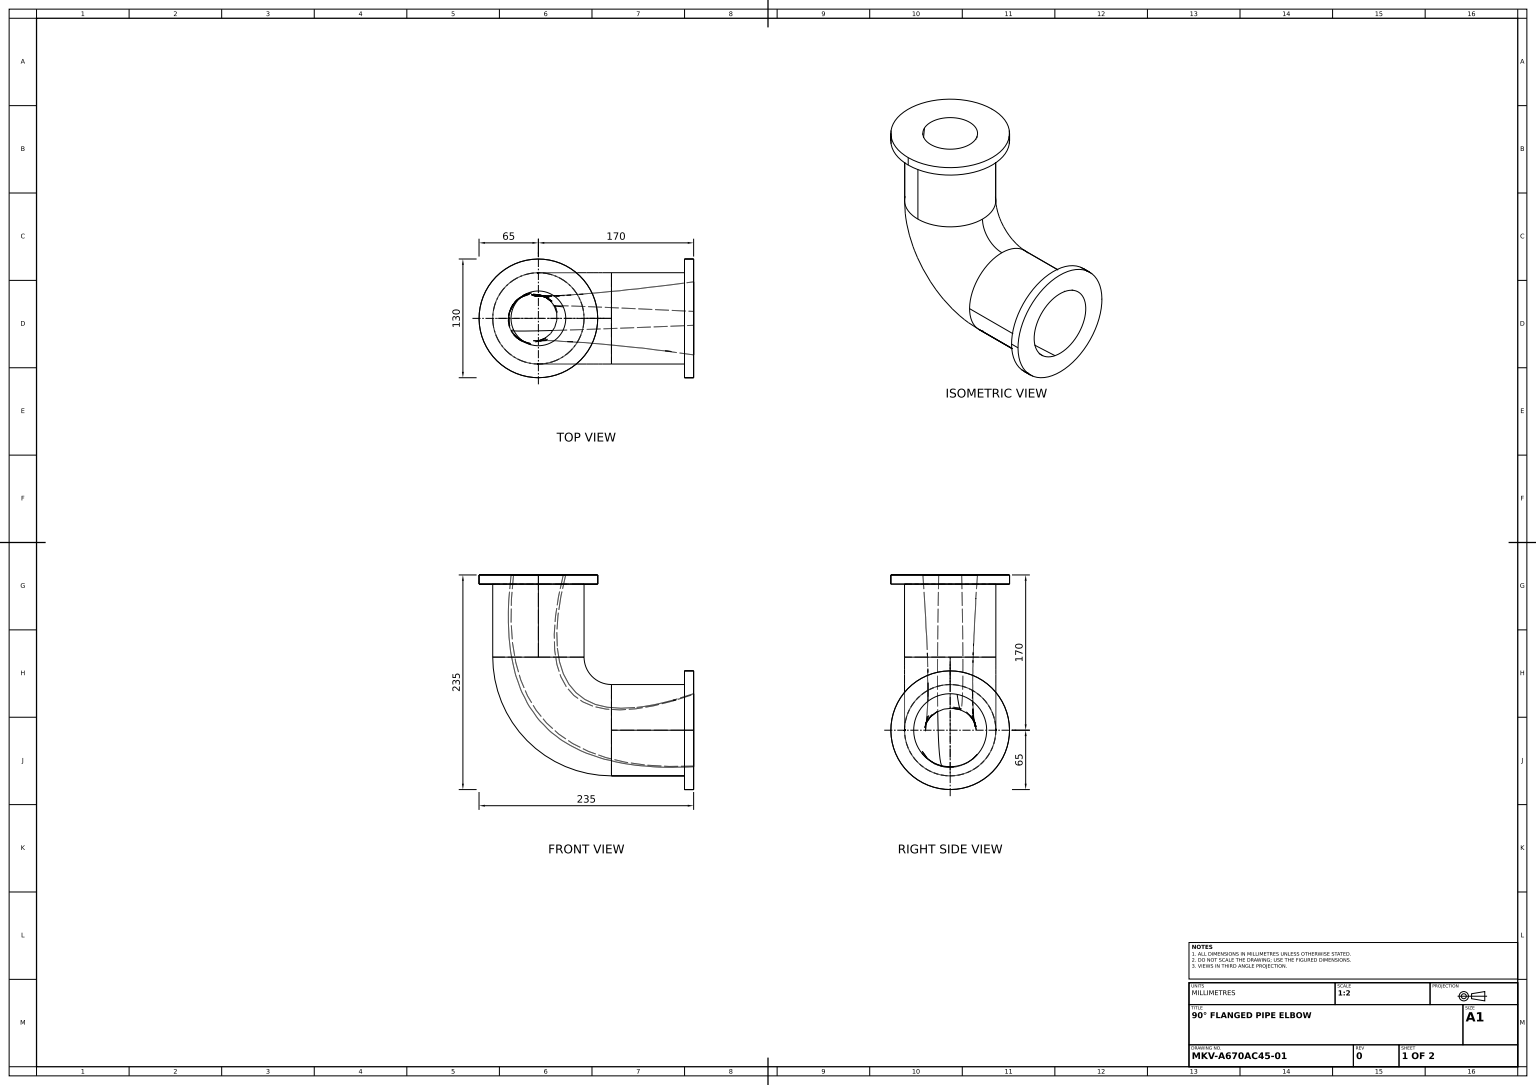
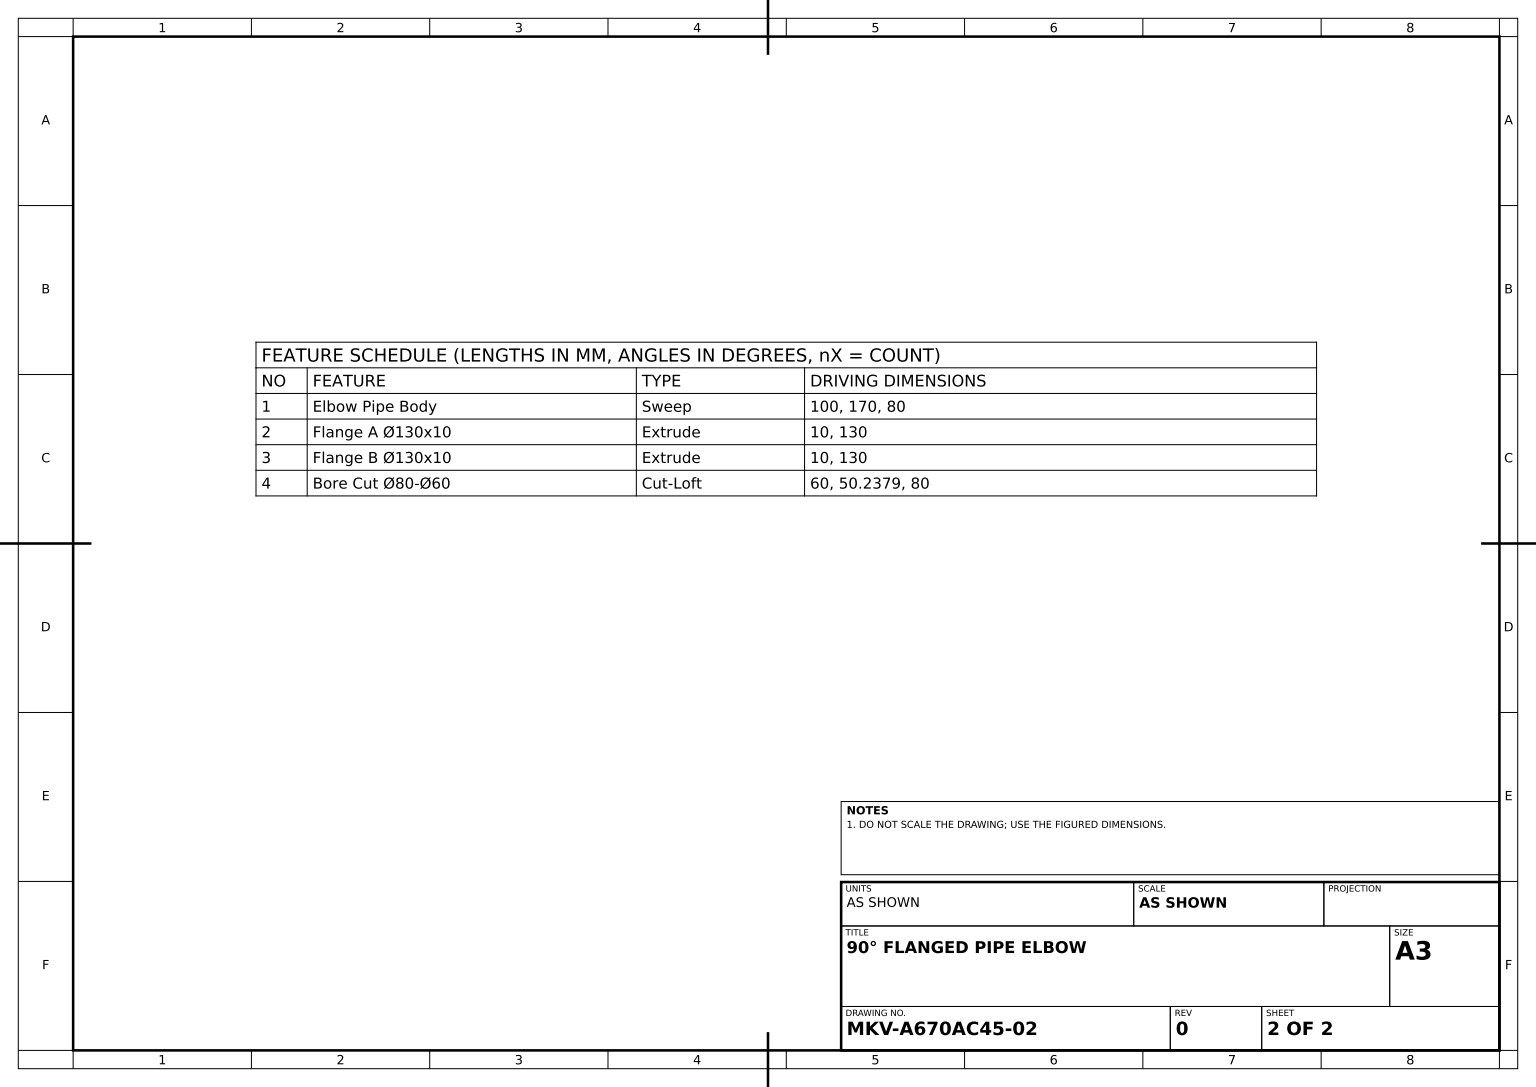
ISO-10303-21;
HEADER;
FILE_DESCRIPTION((''),'2;1');
FILE_NAME('','',(''),(''),'','','');
FILE_SCHEMA(('AUTOMOTIVE_DESIGN'));
ENDSEC;
DATA;
#1=APPLICATION_CONTEXT('');
#2=PRODUCT_CONTEXT('',#1,'mechanical');
#3=PRODUCT('','','',(#2));
#4=PRODUCT_DEFINITION_FORMATION('','',#3);
#5=PRODUCT_DEFINITION_CONTEXT('',#1,'design');
#6=PRODUCT_DEFINITION('','',#4,#5);
#7=PRODUCT_DEFINITION_SHAPE('','',#6);
#8=(LENGTH_UNIT()NAMED_UNIT(*)SI_UNIT(.MILLI.,.METRE.));
#9=(NAMED_UNIT(*)PLANE_ANGLE_UNIT()SI_UNIT($,.RADIAN.));
#10=(NAMED_UNIT(*)SI_UNIT($,.STERADIAN.)SOLID_ANGLE_UNIT());
#11=UNCERTAINTY_MEASURE_WITH_UNIT(LENGTH_MEASURE(1.E-05),#8,'distance_accuracy_value','');
#12=(GEOMETRIC_REPRESENTATION_CONTEXT(3)GLOBAL_UNCERTAINTY_ASSIGNED_CONTEXT((#11))GLOBAL_UNIT_ASSIGNED_CONTEXT((#8,#9,#10))REPRESENTATION_CONTEXT('',''));
#13=CARTESIAN_POINT('',(-170.,170.,65.));
#14=VERTEX_POINT('',#13);
#15=CARTESIAN_POINT('',(-170.,170.,-65.));
#16=VERTEX_POINT('',#15);
#17=CARTESIAN_POINT('',(-170.,170.,0.));
#18=DIRECTION('',(0.,1.,0.));
#19=DIRECTION('',(0.,0.,1.));
#20=AXIS2_PLACEMENT_3D('',#17,#18,#19);
#21=CIRCLE('',#20,65.);
#22=EDGE_CURVE('',#14,#16,#21,.T.);
#23=ORIENTED_EDGE('',*,*,#22,.T.);
#24=EDGE_CURVE('',#16,#14,#21,.T.);
#25=ORIENTED_EDGE('',*,*,#24,.T.);
#26=EDGE_LOOP('',(#23,#25));
#27=FACE_OUTER_BOUND('',#26,.T.);
#28=CARTESIAN_POINT('',(-197.232446,170.,12.585464));
#29=VERTEX_POINT('',#28);
#30=CARTESIAN_POINT('',(-142.767554,170.,-12.585464));
#31=VERTEX_POINT('',#30);
#32=CIRCLE('',#20,30.);
#33=EDGE_CURVE('',#29,#31,#32,.T.);
#34=ORIENTED_EDGE('',*,*,#33,.F.);
#35=EDGE_CURVE('',#31,#29,#32,.T.);
#36=ORIENTED_EDGE('',*,*,#35,.F.);
#37=EDGE_LOOP('',(#34,#36));
#38=FACE_BOUND('',#37,.T.);
#39=PLANE('',#20);
#40=ADVANCED_FACE('',(#27,#38),#39,.T.);
#41=CARTESIAN_POINT('',(-170.,160.,-65.));
#42=VERTEX_POINT('',#41);
#43=CARTESIAN_POINT('',(-170.,160.,65.));
#44=VERTEX_POINT('',#43);
#45=CARTESIAN_POINT('',(-170.,160.,0.));
#46=AXIS2_PLACEMENT_3D('',#45,#18,#19);
#47=CIRCLE('',#46,65.);
#48=EDGE_CURVE('',#42,#44,#47,.T.);
#49=ORIENTED_EDGE('',*,*,#48,.T.);
#50=VECTOR('',#18,1000.);
#51=LINE('',#43,#50);
#52=EDGE_CURVE('',#44,#14,#51,.T.);
#53=ORIENTED_EDGE('',*,*,#52,.T.);
#54=ORIENTED_EDGE('',*,*,#24,.F.);
#55=LINE('',#41,#50);
#56=EDGE_CURVE('',#42,#16,#55,.T.);
#57=ORIENTED_EDGE('',*,*,#56,.F.);
#58=EDGE_LOOP('',(#49,#53,#54,#57));
#59=FACE_OUTER_BOUND('',#58,.T.);
#60=CYLINDRICAL_SURFACE('',#46,65.);
#61=ADVANCED_FACE('',(#59),#60,.T.);
#62=ORIENTED_EDGE('',*,*,#22,.F.);
#63=ORIENTED_EDGE('',*,*,#52,.F.);
#64=EDGE_CURVE('',#44,#42,#47,.T.);
#65=ORIENTED_EDGE('',*,*,#64,.T.);
#66=ORIENTED_EDGE('',*,*,#56,.T.);
#67=EDGE_LOOP('',(#62,#63,#65,#66));
#68=FACE_OUTER_BOUND('',#67,.T.);
#69=ADVANCED_FACE('',(#68),#60,.T.);
#70=CARTESIAN_POINT('',(0.,39.272528,-7.593979));
#71=VERTEX_POINT('',#70);
#72=CARTESIAN_POINT('',(-159.156042,104.12626,-14.002019));
#73=CARTESIAN_POINT('',(-151.137946,15.902503,-14.565282));
#74=CARTESIAN_POINT('',(-63.977673,16.974613,-10.674363));
#75=B_SPLINE_CURVE_WITH_KNOTS('',3,(#30,#72,#73,#74,#70),.UNSPECIFIED.,.F.,.F.,(4,1,4),(0.,0.497690593,1.),.UNSPECIFIED.);
#76=EDGE_CURVE('',#31,#71,#75,.T.);
#77=ORIENTED_EDGE('',*,*,#76,.F.);
#78=ORIENTED_EDGE('',*,*,#35,.T.);
#79=CARTESIAN_POINT('',(0.,-39.272528,7.593979));
#80=VERTEX_POINT('',#79);
#81=CARTESIAN_POINT('',(-205.914144,96.731109,13.989567));
#82=CARTESIAN_POINT('',(-182.354184,-10.749397,14.577735));
#83=CARTESIAN_POINT('',(-74.425847,-42.78391,10.66191));
#84=B_SPLINE_CURVE_WITH_KNOTS('',3,(#28,#81,#82,#83,#79),.UNSPECIFIED.,.F.,.F.,(4,1,4),(0.,0.497690593,1.),.UNSPECIFIED.);
#85=EDGE_CURVE('',#29,#80,#84,.T.);
#86=ORIENTED_EDGE('',*,*,#85,.T.);
#87=CARTESIAN_POINT('',(0.,0.,0.));
#88=DIRECTION('',(1.,0.,0.));
#89=DIRECTION('',(0.,0.,-1.));
#90=AXIS2_PLACEMENT_3D('',#87,#88,#89);
#91=CIRCLE('',#90,40.);
#92=EDGE_CURVE('',#80,#71,#91,.T.);
#93=ORIENTED_EDGE('',*,*,#92,.T.);
#94=EDGE_LOOP('',(#77,#78,#86,#93));
#95=FACE_OUTER_BOUND('',#94,.T.);
#96=CARTESIAN_POINT('',(-142.420249,170.,-11.833964));
#97=CARTESIAN_POINT('',(-158.802751,104.261535,-13.415795));
#98=CARTESIAN_POINT('',(-150.850956,16.223105,-14.091002));
#99=CARTESIAN_POINT('',(-63.856547,17.249974,-9.866034));
#100=CARTESIAN_POINT('',(0.,39.48209,-6.510224));
#101=CARTESIAN_POINT('',(-141.793184,170.,-10.316905));
#102=CARTESIAN_POINT('',(-158.155236,104.524001,-12.226031));
#103=CARTESIAN_POINT('',(-150.318363,16.826305,-13.114681));
#104=CARTESIAN_POINT('',(-63.626177,17.730049,-8.245764));
#105=CARTESIAN_POINT('',(0.,39.809283,-4.346089));
#106=CARTESIAN_POINT('',(-141.051444,170.,-8.009421));
#107=CARTESIAN_POINT('',(-157.359065,104.883527,-10.386657));
#108=CARTESIAN_POINT('',(-149.637653,17.624828,-11.590912));
#109=CARTESIAN_POINT('',(-63.32477,18.238428,-5.795047));
#110=CARTESIAN_POINT('',(0.,40.032464,-1.122111));
#111=CARTESIAN_POINT('',(-140.504777,170.,-5.68032));
#112=CARTESIAN_POINT('',(-156.73494,105.211013,-8.504853));
#113=CARTESIAN_POINT('',(-149.074905,18.315267,-10.011831));
#114=CARTESIAN_POINT('',(-63.065356,18.542261,-3.33961));
#115=CARTESIAN_POINT('',(0.,39.996214,2.067543));
#116=CARTESIAN_POINT('',(-138.372537,170.,8.362294));
#117=CARTESIAN_POINT('',(-154.012519,106.981321,2.9913));
#118=CARTESIAN_POINT('',(-146.39642,21.821688,-0.261243));
#119=CARTESIAN_POINT('',(-61.756394,19.149852,11.367279));
#120=CARTESIAN_POINT('',(0.,38.271208,20.926913));
#121=CARTESIAN_POINT('',(-145.39054,170.,21.675561));
#122=CARTESIAN_POINT('',(-159.333782,106.969125,15.038387));
#123=CARTESIAN_POINT('',(-149.396603,19.850627,10.779144));
#124=CARTESIAN_POINT('',(-62.701043,10.719792,24.554295));
#125=CARTESIAN_POINT('',(0.,24.934057,35.919543));
#126=CARTESIAN_POINT('',(-172.444532,170.,34.178552));
#127=CARTESIAN_POINT('',(-182.904783,103.498668,28.969855));
#128=CARTESIAN_POINT('',(-164.885304,6.92329,25.249978));
#129=CARTESIAN_POINT('',(-67.573902,-19.798698,35.135094));
#130=CARTESIAN_POINT('',(0.,-14.081119,43.463759));
#131=CARTESIAN_POINT('',(-190.286339,170.,27.615459));
#132=CARTESIAN_POINT('',(-198.888059,99.178533,26.054389));
#133=CARTESIAN_POINT('',(-176.459345,-4.148847,23.612691));
#134=CARTESIAN_POINT('',(-72.275785,-37.394329,27.391457));
#135=CARTESIAN_POINT('',(0.,-35.081297,29.269077));
#136=CARTESIAN_POINT('',(-204.178552,170.,-2.444532));
#137=CARTESIAN_POINT('',(-212.940229,94.283685,1.924745));
#138=CARTESIAN_POINT('',(-188.249023,-17.349947,5.54278));
#139=CARTESIAN_POINT('',(-76.575908,-48.173492,-6.067636));
#140=CARTESIAN_POINT('',(0.,-43.463759,-14.081119));
#141=CARTESIAN_POINT('',(-197.615459,170.,-20.286339));
#142=CARTESIAN_POINT('',(-208.395625,93.708972,-13.634341));
#143=CARTESIAN_POINT('',(-185.830754,-16.30736,-8.97525));
#144=CARTESIAN_POINT('',(-76.174149,-39.780058,-23.627757));
#145=CARTESIAN_POINT('',(0.,-29.269077,-35.081297));
#146=CARTESIAN_POINT('',(-170.561467,170.,-32.789331));
#147=CARTESIAN_POINT('',(-184.870898,96.9668,-27.27311));
#148=CARTESIAN_POINT('',(-170.197708,-3.226559,-23.832616));
#149=CARTESIAN_POINT('',(-71.545523,-9.354751,-33.726476));
#150=CARTESIAN_POINT('',(0.,9.746099,-42.625513));
#151=CARTESIAN_POINT('',(-155.873939,170.,-29.507266));
#152=CARTESIAN_POINT('',(-171.810673,100.126758,-26.508706));
#153=CARTESIAN_POINT('',(-160.848905,5.695041,-24.215938));
#154=CARTESIAN_POINT('',(-67.884388,5.253598,-29.297169));
#155=CARTESIAN_POINT('',(0.,27.710987,-33.685638));
#156=CARTESIAN_POINT('',(-146.5604,170.,-18.783486));
#157=CARTESIAN_POINT('',(-162.894714,102.838906,-18.710501));
#158=CARTESIAN_POINT('',(-154.073605,12.735393,-18.30241));
#159=CARTESIAN_POINT('',(-65.188173,13.734283,-17.407276));
#160=CARTESIAN_POINT('',(0.,36.342295,-16.82883));
#161=CARTESIAN_POINT('',(-145.140737,170.,-16.857841));
#162=CARTESIAN_POINT('',(-161.519024,103.282174,-17.27874));
#163=CARTESIAN_POINT('',(-153.013016,13.856377,-17.188998));
#164=CARTESIAN_POINT('',(-64.758355,14.992,-15.29536));
#165=CARTESIAN_POINT('',(0.,37.565013,-13.882618));
#166=CARTESIAN_POINT('',(-143.863949,170.,-14.797629));
#167=CARTESIAN_POINT('',(-160.261913,103.712351,-15.715103));
#168=CARTESIAN_POINT('',(-152.027136,14.918554,-15.950787));
#169=CARTESIAN_POINT('',(-64.352934,16.085765,-13.054959));
#170=CARTESIAN_POINT('',(0.,38.559799,-10.807842));
#171=CARTESIAN_POINT('',(-143.11486,170.,-13.336963));
#172=CARTESIAN_POINT('',(-159.509333,103.990985,-14.588244));
#173=CARTESIAN_POINT('',(-151.424937,15.581902,-15.039562));
#174=CARTESIAN_POINT('',(-64.098799,16.699251,-11.482692));
#175=CARTESIAN_POINT('',(0.,39.062967,-8.677734));
#176=B_SPLINE_SURFACE_WITH_KNOTS('',3,3,((#30,#72,#73,#74,#70),(#96,#97,#98,#99,#100),(#101,#102,#103,#104,#105),(#106,#107,#108,#109,#110),(#111,#112,#113,#114,#115),(#116,#117,#118,#119,#120),(#121,#122,#123,#124,#125),(#126,#127,#128,#129,#130),(#131,#132,#133,#134,#135),(#136,#137,#138,#139,#140),(#141,#142,#143,#144,#145),(#146,#147,#148,#149,#150),(#151,#152,#153,#154,#155),(#156,#157,#158,#159,#160),(#161,#162,#163,#164,#165),(#166,#167,#168,#169,#170),(#171,#172,#173,#174,#175),(#30,#72,#73,#74,#70)),.UNSPECIFIED.,.T.,.F.,.F.,(4,1,1,1,1,2,2,2,1,1,1,1,4),(4,1,4),(0.,0.0125,0.025,0.0375,0.05,0.25,0.5,0.75,0.95,0.9625,0.975,0.9875,1.),(0.,0.497690593,1.),.UNSPECIFIED.);
#177=ADVANCED_FACE('',(#95),#176,.F.);
#178=CARTESIAN_POINT('',(-10.,0.,-50.));
#179=VERTEX_POINT('',#178);
#180=CARTESIAN_POINT('',(-90.,0.,-50.));
#181=VERTEX_POINT('',#180);
#182=CARTESIAN_POINT('',(0.,0.,-50.));
#183=DIRECTION('',(-1.,0.,0.));
#184=VECTOR('',#183,1000.);
#185=LINE('',#182,#184);
#186=EDGE_CURVE('',#179,#181,#185,.T.);
#187=ORIENTED_EDGE('',*,*,#186,.F.);
#188=CARTESIAN_POINT('',(-10.,0.,50.));
#189=VERTEX_POINT('',#188);
#190=CARTESIAN_POINT('',(-10.,0.,0.));
#191=AXIS2_PLACEMENT_3D('',#190,#183,#89);
#192=CIRCLE('',#191,50.);
#193=EDGE_CURVE('',#179,#189,#192,.T.);
#194=ORIENTED_EDGE('',*,*,#193,.T.);
#195=CARTESIAN_POINT('',(-90.,0.,50.));
#196=VERTEX_POINT('',#195);
#197=CARTESIAN_POINT('',(0.,0.,50.));
#198=LINE('',#197,#184);
#199=EDGE_CURVE('',#189,#196,#198,.T.);
#200=ORIENTED_EDGE('',*,*,#199,.T.);
#201=CARTESIAN_POINT('',(-90.,-50.,0.));
#202=VERTEX_POINT('',#201);
#203=CARTESIAN_POINT('',(-90.,0.,0.));
#204=AXIS2_PLACEMENT_3D('',#203,#183,#19);
#205=CIRCLE('',#204,50.);
#206=EDGE_CURVE('',#202,#196,#205,.T.);
#207=ORIENTED_EDGE('',*,*,#206,.F.);
#208=EDGE_CURVE('',#181,#202,#205,.T.);
#209=ORIENTED_EDGE('',*,*,#208,.F.);
#210=EDGE_LOOP('',(#187,#194,#200,#207,#209));
#211=FACE_OUTER_BOUND('',#210,.T.);
#212=AXIS2_PLACEMENT_3D('',#87,#183,#19);
#213=CYLINDRICAL_SURFACE('',#212,50.);
#214=ADVANCED_FACE('',(#211),#213,.T.);
#215=CARTESIAN_POINT('',(-220.,80.,0.));
#216=VERTEX_POINT('',#215);
#217=CARTESIAN_POINT('',(-170.,80.,50.));
#218=VERTEX_POINT('',#217);
#219=CARTESIAN_POINT('',(-170.,80.,0.));
#220=AXIS2_PLACEMENT_3D('',#219,#18,#19);
#221=CIRCLE('',#220,50.);
#222=EDGE_CURVE('',#216,#218,#221,.T.);
#223=ORIENTED_EDGE('',*,*,#222,.F.);
#224=CARTESIAN_POINT('',(-90.,80.,0.));
#225=AXIS2_PLACEMENT_3D('',#224,#89,#183);
#226=CIRCLE('',#225,130.);
#227=EDGE_CURVE('',#202,#216,#226,.T.);
#228=ORIENTED_EDGE('',*,*,#227,.F.);
#229=ORIENTED_EDGE('',*,*,#206,.T.);
#230=CARTESIAN_POINT('',(-90.,50.,0.));
#231=VERTEX_POINT('',#230);
#232=EDGE_CURVE('',#196,#231,#205,.T.);
#233=ORIENTED_EDGE('',*,*,#232,.T.);
#234=CARTESIAN_POINT('',(-120.,80.,0.));
#235=VERTEX_POINT('',#234);
#236=CIRCLE('',#225,30.);
#237=EDGE_CURVE('',#231,#235,#236,.T.);
#238=ORIENTED_EDGE('',*,*,#237,.T.);
#239=EDGE_CURVE('',#218,#235,#221,.T.);
#240=ORIENTED_EDGE('',*,*,#239,.F.);
#241=EDGE_LOOP('',(#223,#228,#229,#233,#238,#240));
#242=FACE_OUTER_BOUND('',#241,.T.);
#243=TOROIDAL_SURFACE('',#225,80.,50.);
#244=ADVANCED_FACE('',(#242),#243,.T.);
#245=ORIENTED_EDGE('',*,*,#237,.F.);
#246=EDGE_CURVE('',#231,#181,#205,.T.);
#247=ORIENTED_EDGE('',*,*,#246,.T.);
#248=ORIENTED_EDGE('',*,*,#208,.T.);
#249=ORIENTED_EDGE('',*,*,#227,.T.);
#250=CARTESIAN_POINT('',(-170.,80.,-50.));
#251=VERTEX_POINT('',#250);
#252=EDGE_CURVE('',#251,#216,#221,.T.);
#253=ORIENTED_EDGE('',*,*,#252,.F.);
#254=EDGE_CURVE('',#235,#251,#221,.T.);
#255=ORIENTED_EDGE('',*,*,#254,.F.);
#256=EDGE_LOOP('',(#245,#247,#248,#249,#253,#255));
#257=FACE_OUTER_BOUND('',#256,.T.);
#258=ADVANCED_FACE('',(#257),#243,.T.);
#259=EDGE_CURVE('',#71,#80,#91,.T.);
#260=ORIENTED_EDGE('',*,*,#259,.T.);
#261=ORIENTED_EDGE('',*,*,#85,.F.);
#262=ORIENTED_EDGE('',*,*,#33,.T.);
#263=ORIENTED_EDGE('',*,*,#76,.T.);
#264=EDGE_LOOP('',(#260,#261,#262,#263));
#265=FACE_OUTER_BOUND('',#264,.T.);
#266=ADVANCED_FACE('',(#265),#176,.F.);
#267=ORIENTED_EDGE('',*,*,#259,.F.);
#268=ORIENTED_EDGE('',*,*,#92,.F.);
#269=EDGE_LOOP('',(#267,#268));
#270=FACE_BOUND('',#269,.T.);
#271=CARTESIAN_POINT('',(0.,0.,65.));
#272=VERTEX_POINT('',#271);
#273=CARTESIAN_POINT('',(0.,0.,-65.));
#274=VERTEX_POINT('',#273);
#275=CIRCLE('',#90,65.);
#276=EDGE_CURVE('',#272,#274,#275,.T.);
#277=ORIENTED_EDGE('',*,*,#276,.T.);
#278=EDGE_CURVE('',#274,#272,#275,.T.);
#279=ORIENTED_EDGE('',*,*,#278,.T.);
#280=EDGE_LOOP('',(#277,#279));
#281=FACE_OUTER_BOUND('',#280,.T.);
#282=PLANE('',#212);
#283=ADVANCED_FACE('',(#270,#281),#282,.F.);
#284=ORIENTED_EDGE('',*,*,#48,.F.);
#285=ORIENTED_EDGE('',*,*,#64,.F.);
#286=EDGE_LOOP('',(#284,#285));
#287=FACE_OUTER_BOUND('',#286,.T.);
#288=CARTESIAN_POINT('',(-170.,160.,-50.));
#289=VERTEX_POINT('',#288);
#290=CARTESIAN_POINT('',(-170.,160.,50.));
#291=VERTEX_POINT('',#290);
#292=DIRECTION('',(0.,-1.,0.));
#293=AXIS2_PLACEMENT_3D('',#45,#292,#19);
#294=CIRCLE('',#293,50.);
#295=EDGE_CURVE('',#289,#291,#294,.T.);
#296=ORIENTED_EDGE('',*,*,#295,.F.);
#297=EDGE_CURVE('',#291,#289,#294,.T.);
#298=ORIENTED_EDGE('',*,*,#297,.F.);
#299=EDGE_LOOP('',(#296,#298));
#300=FACE_BOUND('',#299,.T.);
#301=PLANE('',#46);
#302=ADVANCED_FACE('',(#287,#300),#301,.F.);
#303=ORIENTED_EDGE('',*,*,#193,.F.);
#304=EDGE_CURVE('',#189,#179,#192,.T.);
#305=ORIENTED_EDGE('',*,*,#304,.F.);
#306=EDGE_LOOP('',(#303,#305));
#307=FACE_BOUND('',#306,.T.);
#308=CARTESIAN_POINT('',(-10.,0.,-65.));
#309=VERTEX_POINT('',#308);
#310=CARTESIAN_POINT('',(-10.,0.,65.));
#311=VERTEX_POINT('',#310);
#312=AXIS2_PLACEMENT_3D('',#190,#88,#89);
#313=CIRCLE('',#312,65.);
#314=EDGE_CURVE('',#309,#311,#313,.T.);
#315=ORIENTED_EDGE('',*,*,#314,.F.);
#316=EDGE_CURVE('',#311,#309,#313,.T.);
#317=ORIENTED_EDGE('',*,*,#316,.F.);
#318=EDGE_LOOP('',(#315,#317));
#319=FACE_OUTER_BOUND('',#318,.T.);
#320=PLANE('',#312);
#321=ADVANCED_FACE('',(#307,#319),#320,.F.);
#322=VECTOR('',#88,1000.);
#323=LINE('',#308,#322);
#324=EDGE_CURVE('',#309,#274,#323,.T.);
#325=ORIENTED_EDGE('',*,*,#324,.F.);
#326=ORIENTED_EDGE('',*,*,#314,.T.);
#327=LINE('',#310,#322);
#328=EDGE_CURVE('',#311,#272,#327,.T.);
#329=ORIENTED_EDGE('',*,*,#328,.T.);
#330=ORIENTED_EDGE('',*,*,#278,.F.);
#331=EDGE_LOOP('',(#325,#326,#329,#330));
#332=FACE_OUTER_BOUND('',#331,.T.);
#333=CYLINDRICAL_SURFACE('',#312,65.);
#334=ADVANCED_FACE('',(#332),#333,.T.);
#335=LINE('',#250,#50);
#336=EDGE_CURVE('',#251,#289,#335,.T.);
#337=ORIENTED_EDGE('',*,*,#336,.T.);
#338=ORIENTED_EDGE('',*,*,#295,.T.);
#339=LINE('',#217,#50);
#340=EDGE_CURVE('',#218,#291,#339,.T.);
#341=ORIENTED_EDGE('',*,*,#340,.F.);
#342=ORIENTED_EDGE('',*,*,#239,.T.);
#343=ORIENTED_EDGE('',*,*,#254,.T.);
#344=EDGE_LOOP('',(#337,#338,#341,#342,#343));
#345=FACE_OUTER_BOUND('',#344,.T.);
#346=CYLINDRICAL_SURFACE('',#220,50.);
#347=ADVANCED_FACE('',(#345),#346,.T.);
#348=ORIENTED_EDGE('',*,*,#297,.T.);
#349=ORIENTED_EDGE('',*,*,#336,.F.);
#350=ORIENTED_EDGE('',*,*,#252,.T.);
#351=ORIENTED_EDGE('',*,*,#222,.T.);
#352=ORIENTED_EDGE('',*,*,#340,.T.);
#353=EDGE_LOOP('',(#348,#349,#350,#351,#352));
#354=FACE_OUTER_BOUND('',#353,.T.);
#355=ADVANCED_FACE('',(#354),#346,.T.);
#356=ORIENTED_EDGE('',*,*,#186,.T.);
#357=ORIENTED_EDGE('',*,*,#246,.F.);
#358=ORIENTED_EDGE('',*,*,#232,.F.);
#359=ORIENTED_EDGE('',*,*,#199,.F.);
#360=ORIENTED_EDGE('',*,*,#304,.T.);
#361=EDGE_LOOP('',(#356,#357,#358,#359,#360));
#362=FACE_OUTER_BOUND('',#361,.T.);
#363=ADVANCED_FACE('',(#362),#213,.T.);
#364=ORIENTED_EDGE('',*,*,#328,.F.);
#365=ORIENTED_EDGE('',*,*,#316,.T.);
#366=ORIENTED_EDGE('',*,*,#324,.T.);
#367=ORIENTED_EDGE('',*,*,#276,.F.);
#368=EDGE_LOOP('',(#364,#365,#366,#367));
#369=FACE_OUTER_BOUND('',#368,.T.);
#370=ADVANCED_FACE('',(#369),#333,.T.);
#371=CLOSED_SHELL('',(#40,#61,#69,#177,#214,#244,#258,#266,#283,#302,#321,#334,#347,#355,#363,#370));
#372=MANIFOLD_SOLID_BREP('',#371);
#373=ADVANCED_BREP_SHAPE_REPRESENTATION('',(#372),#12);
#374=SHAPE_DEFINITION_REPRESENTATION(#7,#373);
ENDSEC;
END-ISO-10303-21;
